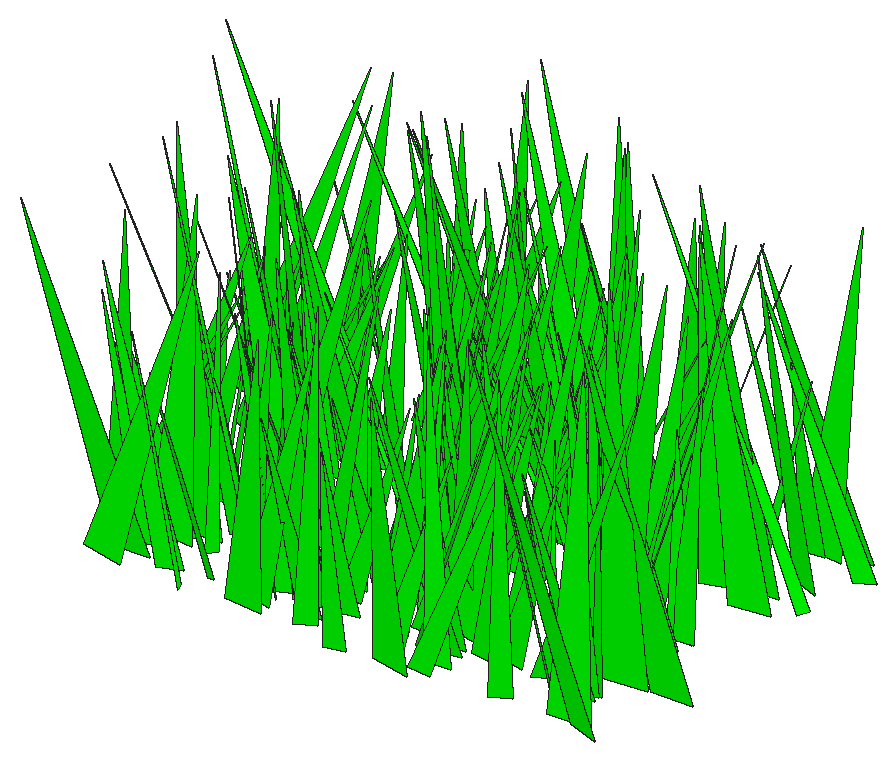
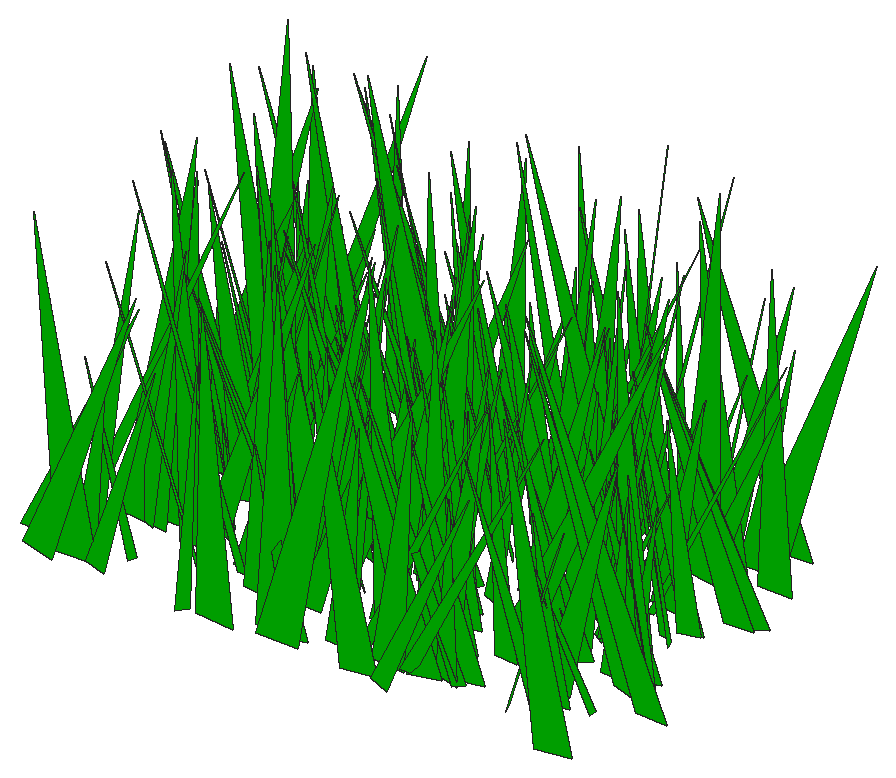
# SketchUp Ruby script. Lengths in inches.
U = 1.inch
M = Sketchup.active_model
def pt(a) = Geom::Point3d.new(a.map { |v| v * U })
def face(e, loops, mat)
  f = e.add_face(loops[0].map { |a| pt(a) })
  loops[1..].each { |l| e.add_face(l.map { |a| pt(a) }).erase! }
  f.material = f.back_material = mat if mat
  f
end
# faces: each face lists its corners as indices into pts; further lists are holes
def faces(e, pts, list, mat = nil) = list.each { |f| face(e, (f[0].is_a?(Array) ? f : [f]).map { |l| l.map { |i| pts[i] } }, mat) }
# xy, xz, yz: faces in a plane at the given z, y or x. An outline is a flat list of corners, or four numbers for a rectangle; further outlines are holes
def ring(l) = l.size == 4 ? [[l[0], l[1]], [l[2], l[1]], [l[2], l[3]], [l[0], l[3]]] : l.each_slice(2).to_a
def flat(e, list, mat, &to3) = list.each { |f| face(e, (f[0].is_a?(Array) ? f : [f]).map { |l| ring(l).map { |u, v| to3.(u, v) } }, mat) }
def xy(e, z, list, mat = nil) = flat(e, list, mat) { |x, y| [x, y, z] }
def xz(e, y, list, mat = nil) = flat(e, list, mat) { |x, z| [x, y, z] }
def yz(e, x, list, mat = nil) = flat(e, list, mat) { |y, z| [x, y, z] }
def lines(e, pts, list) = list.each { |a, b| e.add_line(pt(pts[a]), pt(pts[b])) }
# prism: a flat outline (further loops are holes) pulled along v
def prism(e, loops, v, mat = nil)
  f = face(e, loops, mat); d = Geom::Vector3d.new(v.map { |x| x * U })
  f.pushpull(f.normal.samedirection?(d) ? d.length : -d.length)
end
def box(e, o, s, mat = nil) = prism(e, [[o, [o[0] + s[0], o[1], o[2]], [o[0] + s[0], o[1] + s[1], o[2]], [o[0], o[1] + s[1], o[2]]]], [0, 0, s[2]], mat)
def at(x, y, z, deg = 0) = Geom::Transformation.translation(pt([x, y, z])) * Geom::Transformation.rotation(ORIGIN, Z_AXIS, deg.degrees)
def axes(o, x, y, z) = Geom::Transformation.new([*x, 0, *y, 0, *z, 0, *pt(o).to_a, 1])
def part(name) = M.definitions.add(name)
# library, detail: a bought-in or finely detailed component or shape, given as its bounding box
def library(name, o, s) = part(name).tap { |d| box(d.entities, o, s) }
def detail(e, o, s) = box(e.add_group.entities, o, s)
def put(e, d, t, mat = nil) = e.add_instance(d, t).tap { |i| i.material = mat if mat }
def group(e, t, mat = nil) = e.add_group.tap { |g| g.transformation = t; g.material = mat if mat }.entities
root = M.entities
M.materials.add("[0065_Lime]").color = [0, 255, 0]
c1 = part("fur_instance\#9")
p = [[0.8125,0,1.79],[0.67,-0.02,1.48],[0,-0.11,0],[0,0.11,0]]
faces(c1.entities,p,[[0,1,2,3]])
put(root,c1,axes([91.92,19.48,1.48],[-3.24569,-1.02685,0.182],[7.276,-0.45031,0.71645],[-0.71502,0.07882,6.46446]),"[0065_Lime]")
put(root,c1,axes([92.61,24.42,1.48],[-7.02476,-0.26887,0.02908],[1.8862,-0.97596,-0.89575],[0.32351,-0.148,5.85407]),"[0065_Lime]")
put(root,c1,axes([89.58,28.3,1.48],[4.62409,0.12298,1.08018],[-0.66506,0.67068,-0.67486],[-1.44467,0.08487,3.76811]),"[0065_Lime]")
put(root,c1,axes([89.8,28.16,1.48],[3.69978,-0.35848,0.84872],[2.50533,0.5397,0.41241],[-1.14897,0.02248,3.63218]),"[0065_Lime]")
put(root,c1,axes([91.04,27.25,1.48],[-2.89217,0.42946,0.19512],[-3.00695,-0.40642,0.48535],[0.59731,0.03349,3.3881]),"[0065_Lime]")
put(root,c1,axes([89.41,33.39,1.48],[2.35109,-0.91741,1.43617],[6.76165,0.31301,-0.62389],[0.15009,0.26967,5.60987]),"[0065_Lime]")
put(root,c1,axes([91.9,30.17,1.48],[-2.7268,0.71224,1.12489],[-5.24775,-0.35859,-0.80864],[-0.25507,-0.23663,4.61131]),"[0065_Lime]")
put(root,c1,axes([90.42,20.89,1.48],[-2.77263,-0.88074,1.86179],[6.51417,-0.43273,-0.44095],[1.44572,0.26072,5.55742]),"[0065_Lime]")
put(root,c1,axes([88.35,29.73,1.48],[5.98614,0.89507,0.55434],[-6.40524,0.83845,0.39983],[-0.10668,-0.11712,7.09892]),"[0065_Lime]")
put(root,c1,axes([91.03,28.375,1.48],[1.26403,-0.5368,0.92286],[3.89497,0.20179,0.40328],[-0.84273,0.12746,3.24813]),"[0065_Lime]")
put(root,c1,axes([89.76,27.91,1.48],[3.22694,0.49716,0.9492],[-3.72481,0.43486,0.74612],[-0.07426,-0.20831,3.82301]),"[0065_Lime]")
put(root,c1,axes([92.01,20.15,1.48],[-3.96111,0.47657,1.19406],[-3.61441,-0.56262,-0.40871],[0.77039,-0.18925,4.22195]),"[0065_Lime]")
put(root,c1,axes([92.32,32.04,1.48],[-4.69595,-0.0008,0.64551],[0.12397,-0.66172,0.56935],[0.78386,0.09988,3.77708]),"[0065_Lime]")
put(root,c1,axes([90.81,24.77,1.48],[-2.10896,0.56806,1.28674],[-4.12646,-0.33907,0.54107],[1.34808,-0.14921,3.66919]),"[0065_Lime]")
put(root,c1,axes([92.78,21.3125,1.48],[-3.49706,0.4689,0.33335],[-3.35687,-0.48239,-0.56302],[-0.18611,-0.10996,3.89128]),"[0065_Lime]")
put(root,c1,axes([92.83,26.69,1.48],[-8.75074,-0.02631,1.80702],[-0.08493,-1.25958,-0.88654],[2.22778,-0.15135,7.06419]),"[0065_Lime]")
put(root,c1,axes([90.9,25.63,1.48],[4.04277,0.01574,1.04251],[0.11871,0.58679,-0.60154],[-1.28105,0.10406,3.23424]),"[0065_Lime]")
put(root,c1,axes([92.92,26.6875,1.48],[-3.81514,-0.23371,0.32544],[1.70696,-0.52916,0.50596],[0.11291,0.10271,3.34735]),"[0065_Lime]")
put(root,c1,axes([89.25,23.09,1.48],[5.133,-0.39887,0.1458],[2.83923,0.71551,-0.54425],[0.16811,0.09442,4.74]),"[0065_Lime]")
put(root,c1,axes([94.78,28.57,1.48],[-7.87068,0.70308,0.34183],[-5.02024,-1.0998,-0.67967],[-0.09552,-0.13074,7.55576]),"[0065_Lime]")
put(root,c1,axes([89.88,23.375,1.48],[3.25022,0.81752,0.41828],[-5.82461,0.44758,0.63277],[0.43207,-0.11612,5.38373]),"[0065_Lime]")
put(root,c1,axes([90,30.6,1.48],[4.06266,-0.08517,0.13062],[0.62466,0.56262,-0.56183],[-0.05456,0.09935,3.29362]),"[0065_Lime]")
put(root,c1,axes([91.54,26.5625,1.48],[3.93743,0.99503,1.61528],[-7.17486,0.58923,-0.59105],[-1.615,-0.19181,6.56394]),"[0065_Lime]")
put(root,c1,axes([91.58,26.08,1.48],[4.62297,0.14912,1.48012],[-0.79049,0.6944,-0.71064],[-1.95252,0.07193,3.79218]),"[0065_Lime]")
put(root,c1,axes([89.97,28.9375,1.48],[6.16256,0.78027,0.25446],[-5.49819,0.8646,-0.73643],[-0.83749,0.06533,6.70714]),"[0065_Lime]")
put(root,c1,axes([92.52,23.83,1.48],[0.18841,-0.66559,1.23709],[4.89414,0.06316,0.64558],[-0.89245,0.20587,3.80149]),"[0065_Lime]")
put(root,c1,axes([90.24,32.62,1.48],[4.00656,0.60155,0.63818],[-4.35167,0.55614,0.51018],[-0.07102,-0.14079,4.74197]),"[0065_Lime]")
put(root,c1,axes([91.14,30.91,1.48],[0.02874,-0.59972,0.24403],[4.21195,-0.00344,-0.61147],[0.75158,0.04221,3.41741]),"[0065_Lime]")
put(root,c1,axes([90.77,24.6,1.48],[3.40058,0.61504,0.9237],[-4.51374,0.47364,0.42691],[-0.27052,-0.17163,4.48824]),"[0065_Lime]")
put(root,c1,axes([89.79,22.42,1.48],[5.33353,0.25038,0.28486],[-1.81571,0.73758,0.76943],[-0.02711,-0.14168,4.50888]),"[0065_Lime]")
put(root,c1,axes([91.4,25.32,1.48],[4.15817,-0.09228,0.84533],[0.5224,0.59889,0.49051],[-1.11283,-0.06367,3.38892]),"[0065_Lime]")
put(root,c1,axes([93.59,19.34,1.48],[3.44491,-0.59274,2.93219],[4.61273,0.6373,0.73132],[-3.08396,0.29112,4.36922]),"[0065_Lime]")
put(root,c1,axes([92.99,27.52,1.48],[0.50021,0.56005,0.98968],[-4.05679,0.10481,-0.63089],[-0.95276,-0.15226,3.20588]),"[0065_Lime]")
put(root,c1,axes([92.96,21.65,1.48],[2.47919,1.16013,2.39013],[-8.58156,0.40836,-0.75235],[-1.7761,-0.35368,6.9714]),"[0065_Lime]")
put(root,c1,axes([92.32,20.95,1.48],[-1.36073,1.04462,1.98532],[-7.74686,-0.22878,0.52058],[1.09942,-0.31913,6.12535]),"[0065_Lime]")
put(root,c1,axes([93.99,25.67,1.48],[-5.63766,-0.40911,1.36757],[3.13367,-0.80652,0.46238],[1.21799,0.18139,5.14041]),"[0065_Lime]")
put(root,c1,axes([93.57,27.14,1.48],[0.24656,0.87384,0.72564],[-6.21892,0.05173,-0.68939],[-0.89053,-0.11932,5.01518]),"[0065_Lime]")
put(root,c1,axes([93.65,26.5,1.48],[-7.34357,-0.52266,1.95346],[3.62738,-1.085,-0.7053],[2.53863,0.03841,6.65863]),"[0065_Lime]")
put(root,c1,axes([94.04,22.4375,1.48],[0.02603,-0.59967,1.14393],[4.35653,0.05176,0.84369],[-1.10039,0.19075,3.3673]),"[0065_Lime]")
put(root,c1,axes([91.3125,18.75,1.48],[3.56995,0.98302,0.75879],[-7.048,0.48889,0.71644],[0.36871,-0.17267,6.3482]),"[0065_Lime]")
put(root,c1,axes([94.92,24.03,1.48],[-3.06708,1.05085,0.18006],[-7.46739,-0.42789,-0.48009],[-0.46251,-0.06018,6.55721]),"[0065_Lime]")
put(root,c1,axes([93.96,26.22,1.48],[-0.35939,-0.56633,0.89823],[4.13365,-0.02534,0.55892],[-0.61279,0.1612,3.24348]),"[0065_Lime]")
put(root,c1,axes([96.28,32.16,1.48],[-6.77188,0.27227,0.21489],[-1.95548,-0.94195,-0.7813],[-0.0128,-0.13997,5.67585]),"[0065_Lime]")
put(root,c1,axes([93.1,24.56,1.48],[3.48195,-0.26171,1.27705],[2.25104,0.49277,-0.67705],[-0.9308,0.2127,3.13981]),"[0065_Lime]")
put(root,c1,axes([94.58,18.6,1.48],[-5.3622,-0.02784,1.16169],[0.04171,-0.77552,-0.4953],[1.44123,-0.08112,4.33646]),"[0065_Lime]")
put(root,c1,axes([95,19.66,1.48],[-4.02091,-0.1927,0.537],[1.4559,-0.56336,0.43859],[0.44365,0.10228,3.4277]),"[0065_Lime]")
put(root,c1,axes([92.29,28.17,1.48],[4.68915,-0.38873,0.81739],[2.92828,0.64294,-0.86891],[-0.29672,0.20182,4.34245]),"[0065_Lime]")
put(root,c1,axes([92.98,28.25,1.48],[3.17941,-0.50135,1.25079],[3.87054,0.43291,-0.69516],[-0.33628,0.24265,3.82459]),"[0065_Lime]")
put(root,c1,axes([95.95,20.75,1.48],[-9.06066,0.02591,1.57194],[-0.0697,-1.2997,0.45217],[1.94005,0.07434,7.3577]),"[0065_Lime]")
put(root,c1,axes([93.97,21,1.48],[5.84968,-0.28453,1.8218],[1.88023,0.88016,0.61173],[-2.36242,-0.00402,4.9979]),"[0065_Lime]")
put(root,c1,axes([96.45,33.36,1.48],[-3.92188,-0.48157,0.54721],[3.48617,-0.53123,0.86575],[-0.21028,0.17445,4.14707]),"[0065_Lime]")
put(root,c1,axes([96.13,26.02,1.48],[2.66254,0.7062,3.1752],[-5.72082,0.52604,-0.74642],[-2.78699,-0.40513,4.56559]),"[0065_Lime]")
put(root,c1,axes([94.69,23.99,1.48],[-3.47755,-0.55923,1.54151],[4.09865,-0.53505,-0.38659],[1.62212,0.15303,4.28154]),"[0065_Lime]")
put(root,c1,axes([94.98,31.8125,1.48],[1.89635,0.58542,0.48265],[-4.0538,0.27867,-0.7882],[-1.12956,-0.01729,3.63899]),"[0065_Lime]")
put(root,c1,axes([94.32,29.62,1.48],[3.96928,-0.50861,0.78173],[3.52731,0.57385,0.66095],[-1.25816,0.00424,4.31923]),"[0065_Lime]")
put(root,c1,axes([95.62,31.26,1.48],[-3.60186,-0.89989,0.59524],[6.39015,-0.51395,-0.45239],[0.84485,0.05087,5.95941]),"[0065_Lime]")
put(root,c1,axes([94.9,22.94,1.48],[4.65332,0.1835,1.54487],[-1.66986,0.68285,0.61007],[-1.58872,-0.18026,3.88367]),"[0065_Lime]")
put(root,c1,axes([94.21,31.46,1.48],[1.35391,0.67375,1.23494],[-4.97952,0.14855,0.89635],[0.70629,-0.24421,3.95224]),"[0065_Lime]")
put(root,c1,axes([96.59,23.53,1.48],[-2.92017,0.39625,1.0527],[-3.09301,-0.3915,-0.73886],[0.24508,-0.21949,3.2183]),"[0065_Lime]")
put(root,c1,axes([98.27,31.92,1.48],[-6.97872,0.18079,0.44711],[-1.35547,-0.97103,-0.84115],[0.34673,-0.15718,5.71063]),"[0065_Lime]")
put(root,c1,axes([98.65,21.36,1.48],[-7.58601,-0.24268,0.39256],[1.75768,-1.06469,0.41787],[0.35528,0.08554,6.31464]),"[0065_Lime]")
put(root,c1,axes([95.74,31.46,1.48],[2.89192,-0.97652,1.20471],[7.01807,0.42769,0.47013],[-1.11118,0.15977,6.10459]),"[0065_Lime]")
put(root,c1,axes([97,26.9375,1.48],[-4.809,-0.40122,1.63168],[3.26029,-0.68769,0.69141],[1.24379,0.25134,4.49638]),"[0065_Lime]")
put(root,c1,axes([97.2,28.99,1.48],[-4.79847,-0.58684,0.55181],[4.05876,-0.67916,-0.85042],[1.19503,-0.04971,5.10404]),"[0065_Lime]")
put(root,c1,axes([97.34,20.45,1.48],[3.29526,-0.56739,2.37379],[4.25461,0.5763,0.708],[-2.5921,0.22461,4.17981]),"[0065_Lime]")
put(root,c1,axes([97.23,20.11,1.48],[-8.2028,-0.2169,2.21285],[1.39841,-1.21403,-0.55761],[2.79783,-0.02911,6.76643]),"[0065_Lime]")
put(root,c1,axes([95.75,29.83,1.48],[3.9972,0.6986,0.67111],[-4.93396,0.57262,-0.5301],[-1.0264,-0.03202,5.16178]),"[0065_Lime]")
put(root,c1,axes([94.43,31.84,1.48],[6.13335,-0.25662,0.59584],[1.8984,0.86035,-0.51303],[-0.51748,0.11473,5.18006]),"[0065_Lime]")
put(root,c1,axes([97.01,32.21,1.48],[1.35334,-0.78828,1.09447],[5.68313,0.21554,0.55238],[-0.99121,0.15954,4.66139]),"[0065_Lime]")
put(root,c1,axes([96.17,20.04,1.48],[-3.0635,-0.7169,2.06526],[5.32815,-0.50401,-0.63327],[2.02148,0.24201,4.799]),"[0065_Lime]")
put(root,c1,axes([96.41,28.73,1.48],[-2.88419,-0.55562,1.77818],[4.03701,-0.48056,-0.6993],[2.02893,0.16635,3.91914]),"[0065_Lime]")
put(root,c1,axes([97.02,27.95,1.48],[4.01211,-0.20807,1.20173],[1.31206,0.60007,0.58326],[-1.62906,-0.02915,3.42943]),"[0065_Lime]")
put(root,c1,axes([96.43,29.51,1.48],[4.03494,0.59472,0.31955],[-4.14039,0.56714,-0.77818],[-0.96142,0.05355,4.69237]),"[0065_Lime]")
put(root,c1,axes([95.11,22.55,1.48],[7.41351,-0.70839,1.27092],[5.18238,1.04872,-0.41399],[-0.99944,0.18329,7.28065]),"[0065_Lime]")
put(root,c1,axes([96.41,29.53,1.48],[-0.01607,-0.59195,0.6162],[4.15328,-0.02789,-0.82607],[1.03465,0.10275,3.32558]),"[0065_Lime]")
put(root,c1,axes([98.6,30.34,1.48],[-4.83189,-0.82478,1.6828],[6.17604,-0.68084,0.55145],[0.76717,0.28629,6.1594]),"[0065_Lime]")
put(root,c1,axes([98.72,22.33,1.48],[-5.0712,0.17989,0.7661],[-1.38387,-0.71742,-0.41608],[0.78159,-0.10305,4.234]),"[0065_Lime]")
put(root,c1,axes([96.88,18.93,1.48],[0.07756,-0.90827,0.96952],[6.55338,-0.00216,-0.41461],[0.50402,0.16783,5.24171]),"[0065_Lime]")
put(root,c1,axes([96.87,29.85,1.48],[0.23418,0.58236,1.02324],[-4.30254,0.01099,0.44191],[0.49642,-0.17947,3.34742]),"[0065_Lime]")
put(root,c1,axes([95.63,32.08,1.48],[4.04911,-0.82869,0.45845],[5.91356,0.5596,-0.66201],[0.35608,0.1298,5.78109]),"[0065_Lime]")
put(root,c1,axes([98.43,20.34,1.48],[3.146,0.86777,2.32926],[-6.42121,0.52544,-0.82127],[-2.25938,-0.28503,5.57735]),"[0065_Lime]")
put(root,c1,axes([97.43,27.34,1.48],[-3.77375,0.12988,1.78464],[-0.69374,-0.61272,0.52366],[2.27745,0.02858,3.11667]),"[0065_Lime]")
put(root,c1,axes([97.27,23.65,1.48],[0.06631,0.84537,0.371],[-5.98966,0.00152,0.59219],[0.72509,-0.06475,4.85793]),"[0065_Lime]")
put(root,c1,axes([97.73,30.89,1.48],[3.76272,1.15651,1.00381],[-8.19997,0.54771,-0.80828],[-1.4221,-0.09816,7.31663]),"[0065_Lime]")
put(root,c1,axes([96.86,19.53,1.48],[3.13879,0.7728,1.39934],[-5.76187,0.4247,0.6919],[-0.07946,-0.26944,5.10409]),"[0065_Lime]")
put(root,c1,axes([98.94,19.74,1.48],[-0.671,-0.6326,0.24657],[4.47151,-0.08747,0.53171],[-0.60374,0.05526,3.66397]),"[0065_Lime]")
put(root,c1,axes([99.13,27.23,1.48],[3.53624,1.04666,3.01769],[-7.90001,0.60022,-0.85075],[-2.6143,-0.39801,6.65272]),"[0065_Lime]")
put(root,c1,axes([97.19,27.82,1.48],[2.91879,0.6709,0.89423],[-4.89693,0.40524,0.38767],[-0.15692,-0.16692,4.53533]),"[0065_Lime]")
put(root,c1,axes([99.05,21.11,1.48],[-5.98973,0.45164,2.31292],[-3.83022,-0.87203,-0.85691],[1.93532,-0.32803,5.46246]),"[0065_Lime]")
put(root,c1,axes([97.45,33.16,1.48],[0.67535,0.89881,2.10819],[-6.86108,0.04787,0.7704],[0.74631,-0.3733,5.17481]),"[0065_Lime]")
put(root,c1,axes([99.23,27.38,1.48],[-6.73477,-0.69264,1.98789],[5.01224,-0.99626,-0.3965],[2.26872,0.14488,6.77708]),"[0065_Lime]")
put(root,c1,axes([101,23.42,1.48],[-6.17188,0.12817,0.08532],[-0.89091,-0.86023,0.66272],[0.22201,0.11113,5.03136]),"[0065_Lime]")
put(root,c1,axes([98.13,26.65,1.48],[3.85492,-0.13487,0.78219],[0.83073,0.55564,0.50159],[-1.07511,-0.05426,3.19221]),"[0065_Lime]")
put(root,c1,axes([98.99,32.16,1.48],[1.25087,-0.68207,0.7598],[4.87414,0.19272,0.48801],[-0.8224,0.10479,4.04797]),"[0065_Lime]")
put(root,c1,axes([101.65,29.14,1.48],[-5.65504,-0.91894,0.24835],[6.5208,-0.78557,0.83936],[-0.58275,0.12712,6.98219]),"[0065_Lime]")
put(root,c1,axes([98.76,22.14,1.48],[-1.56191,0.72731,0.5264],[-5.15281,-0.22989,0.52752],[0.81092,-0.05991,4.36593]),"[0065_Lime]")
put(root,c1,axes([100.75,33.14,1.48],[-5.09117,0.98867,0.97003],[-7.12989,-0.71342,-0.3938],[0.3021,-0.1758,7.05329]),"[0065_Lime]")
put(root,c1,axes([99.73,20.54,1.48],[0.21944,-0.71584,1.10892],[5.19335,0.06265,0.67523],[-0.91637,0.18364,4.09229]),"[0065_Lime]")
put(root,c1,axes([99.99,30.3,1.48],[-7.25894,-0.28331,2.29608],[2.47774,-1.06729,0.76994],[2.42774,0.24217,6.07948]),"[0065_Lime]")
put(root,c1,axes([98.27,24.32,1.48],[4.82662,0.10074,0.65315],[-0.53372,0.67411,-0.87433],[-0.9348,0.13524,3.87161]),"[0065_Lime]")
put(root,c1,axes([99.17,19.22,1.48],[6.00487,-0.56016,1.82566],[3.95589,0.89718,0.61538],[-2.29783,0.08071,5.8304]),"[0065_Lime]")
put(root,c1,axes([101.3125,30.86,1.48],[-4.0096,0.58161,0.46494],[-4.17832,-0.55757,-0.46903],[-0.02049,-0.11405,4.66395]),"[0065_Lime]")
put(root,c1,axes([100.71,21.65,1.48],[-0.04136,-0.70623,0.08517],[4.91148,-0.00254,0.87209],[-1.07149,0.01561,3.99418]),"[0065_Lime]")
put(root,c1,axes([98.77,20.62,1.48],[-5.2944,-0.58766,3.22173],[4.40357,-0.90025,-0.71452],[3.71299,0.22973,5.44132]),"[0065_Lime]")
put(root,c1,axes([101.37,30.6875,1.48],[-6.69287,0.05615,1.49717],[-0.71159,-0.95938,-0.89908],[1.74389,-0.17598,5.37914]),"[0065_Lime]")
put(root,c1,axes([102.23,30.4,1.48],[-6.22703,0.97138,0.22501],[-6.88805,-0.87537,0.50627],[0.64738,0.02974,7.55102]),"[0065_Lime]")
put(root,c1,axes([102.09,28.44,1.48],[-4.57817,0.0141,0.06638],[-0.1099,-0.6382,-0.4719],[0.06821,-0.08176,3.69483]),"[0065_Lime]")
put(root,c1,axes([99.29,29.02,1.48],[3.67206,0.71727,1.24036],[-5.31064,0.51348,0.45244],[-0.42237,-0.22023,5.09476]),"[0065_Lime]")
put(root,c1,axes([99.23,21.4,1.48],[3.65346,-0.46943,0.82904],[3.4828,0.50527,-0.56798],[-0.26356,0.16961,3.98661]),"[0065_Lime]")
put(root,c1,axes([100.07,22.29,1.48],[3.58474,0.46932,0.514],[-3.20099,0.5095,-0.81802],[-1.14371,0.04501,3.90049]),"[0065_Lime]")
put(root,c1,axes([97.95,26.51,1.48],[7.68545,-0.19898,0.63195],[1.48887,1.07853,-0.60092],[-0.62611,0.12229,6.3282]),"[0065_Lime]")
put(root,c1,axes([99.55,23.67,1.48],[-3.176,-0.44217,2.04305],[3.05681,-0.55738,-0.89815],[2.62036,0.11429,3.52402]),"[0065_Lime]")
put(root,c1,axes([100.87,18.57,1.48],[1.84091,-0.55287,0.9926],[3.98598,0.28648,0.45583],[-1.04005,0.11935,3.50387]),"[0065_Lime]")
put(root,c1,axes([99.44,26.61,1.48],[7.19532,0.51889,2.065],[-4.08172,1.03739,0.67527],[-1.8494,-0.2708,6.54377]),"[0065_Lime]")
put(root,c1,axes([101.19,32.6,1.48],[-3.44879,1.00705,1.58353],[-7.30548,-0.51427,0.43196],[1.33494,-0.21264,6.45495]),"[0065_Lime]")
put(root,c1,axes([99.52,26.02,1.48],[2.31844,-0.59017,0.22756],[4.14684,0.31254,-0.79284],[0.7224,0.1,3.82088]),"[0065_Lime]")
put(root,c1,axes([100.26,32.76,1.48],[0.23878,-0.54852,1.10261],[4.03808,-0.00953,-0.73744],[0.87721,0.19317,3.09452]),"[0065_Lime]")
put(root,c1,axes([101.77,22.9,1.48],[-0.23271,0.92191,0.64966],[-6.58665,-0.02307,-0.46413],[-0.54624,-0.1146,5.31981]),"[0065_Lime]")
put(root,c1,axes([100.68,22.49,1.48],[-0.01571,0.81854,1.26315],[-5.99652,-0.0246,0.48491],[0.62112,-0.21683,4.7134]),"[0065_Lime]")
put(root,c1,axes([102.65,28.29,1.48],[-5.45352,-0.84059,1.64861],[6.24494,-0.77393,0.44529],[0.94529,0.26341,6.56935]),"[0065_Lime]")
put(root,c1,axes([102.05,25.9375,1.48],[-1.10696,0.691,0.74359],[-4.99459,-0.14565,-0.38414],[-0.26837,-0.13958,4.08205]),"[0065_Lime]")
put(root,c1,axes([100.7,28.83,1.48],[3.97803,0.16264,0.42914],[-1.02369,0.55382,-0.75481],[-0.75504,0.10603,3.28435]),"[0065_Lime]")
put(root,c1,axes([101.12,24.09,1.48],[3.49977,0.40202,0.29265],[-2.73845,0.48829,-0.80898],[-0.90318,0.07733,3.58684]),"[0065_Lime]")
put(root,c1,axes([100.14,24.06,1.48],[8.62324,0.16471,1.72476],[-1.32436,1.24285,0.40388],[-2.02881,-0.11122,7.06723]),"[0065_Lime]")
put(root,c1,axes([102.42,23.2,1.48],[0.08837,0.68836,0.95847],[-5.00202,0.03187,-0.46173],[-0.60484,-0.16296,3.9585]),"[0065_Lime]")
put(root,c1,axes([102.05,27.11,1.48],[2.39831,0.50673,0.09199],[-3.48865,0.33057,-0.839],[-0.91997,0.06744,3.42139]),"[0065_Lime]")
put(root,c1,axes([101.91,21.8,1.48],[5.97637,-0.22166,2.131],[2.01129,0.89367,-0.61718],[-2.3036,0.2052,4.98972]),"[0065_Lime]")
put(root,c1,axes([104.02,20.55,1.48],[-4.01416,-0.57477,0.89186],[4.23475,-0.54402,0.86265],[-0.01595,0.21434,4.58118]),"[0065_Lime]")
put(root,c1,axes([104.14,27.9,1.48],[-3.83485,-0.3415,0.30394],[2.4501,-0.52249,0.78146],[-0.20754,0.14188,3.60935]),"[0065_Lime]")
put(root,c1,axes([101.45,20.75,1.48],[3.47663,0.85199,1.53017],[-6.33236,0.4868,0.43673],[-0.45062,-0.2675,5.66837]),"[0065_Lime]")
put(root,c1,axes([102.85,31.16,1.48],[2.66331,1.05933,1.93104],[-7.76446,0.41647,-0.57031],[-1.47735,-0.27909,6.47852]),"[0065_Lime]")
put(root,c1,axes([103.07,22.67,1.48],[-2.58882,-0.63951,0.23267],[4.49639,-0.36569,-0.5787],[0.75944,-0.01489,4.21943]),"[0065_Lime]")
put(root,c1,axes([102.38,30.65,1.48],[-5.38241,-0.84504,2.57452],[6.14859,-0.84719,-0.81288],[2.89445,0.22825,6.51426]),"[0065_Lime]")
put(root,c1,axes([102.98,18.74,1.48],[-2.03752,-0.92539,0.12117],[6.53216,-0.28667,-0.68636],[0.84999,-0.01521,5.56513]),"[0065_Lime]")
put(root,c1,axes([103.67,20.98,1.48],[-0.73871,-0.74986,1.05637],[5.47816,-0.08747,0.4541],[-0.39172,0.19086,4.35849]),"[0065_Lime]")
put(root,c1,axes([103.39,30.36,1.48],[2.63272,0.94834,1.65151],[-6.87582,0.41247,-0.68443],[-1.54698,-0.21937,5.85268]),"[0065_Lime]")
put(root,c1,axes([102.07,20,1.48],[1.69388,0.64425,0.27951],[-4.58141,0.23219,0.43676],[0.38655,-0.07123,3.95168]),"[0065_Lime]")
put(root,c1,axes([102.21,25.03,1.48],[2.94807,0.53939,0.99148],[-4.01448,0.41061,0.41249],[-0.3236,-0.17985,3.91529]),"[0065_Lime]")
put(root,c1,axes([104.24,30.24,1.48],[-0.74997,0.68554,1.17064],[-5.0122,-0.06478,-0.85336],[-0.86644,-0.21865,3.92327]),"[0065_Lime]")
put(root,c1,axes([103.4375,27.51,1.48],[-3.62563,0.37105,1.13579],[-2.61389,-0.54346,0.42857],[1.44575,-0.05204,3.62316]),"[0065_Lime]")
put(root,c1,axes([103.22,21.95,1.48],[-3.49713,-0.76158,1.86047],[5.56833,-0.54914,-0.60715],[1.89722,0.20791,5.21137]),"[0065_Lime]")
put(root,c1,axes([103.07,33.4,1.48],[2.92682,-0.92936,0.13218],[6.57981,0.41151,0.55511],[-0.6897,-0.01803,5.85679]),"[0065_Lime]")
put(root,c1,axes([102.76,28.42,1.48],[0.80048,0.95404,1.60072],[-7.03915,0.08206,0.69027],[0.64835,-0.28703,5.51791]),"[0065_Lime]")
put(root,c1,axes([104.07,19.79,1.48],[5.12374,-0.48293,2.99449],[4.27694,0.8069,-0.48145],[-2.65927,0.36727,4.99529]),"[0065_Lime]")
put(root,c1,axes([104.32,33.46,1.48],[-5.14227,0.32701,1.34956],[-2.16441,-0.75897,0.70592],[1.86653,0.02082,4.53661]),"[0065_Lime]")
put(root,c1,axes([102.2,25.97,1.48],[5.08179,0.57849,0.57673],[-4.17316,0.7101,0.46202],[-0.1892,-0.12486,5.2997]),"[0065_Lime]")
put(root,c1,axes([102.77,20.38,1.48],[6.3305,0.05353,0.87463],[-0.24876,0.89626,-0.64688],[-1.1133,0.10413,5.11791]),"[0065_Lime]")
put(root,c1,axes([103.16,21.8,1.48],[2.1432,1.21374,1.30258],[-8.77271,0.28356,0.69655],[0.46061,-0.24683,7.2054]),"[0065_Lime]")
put(root,c1,axes([101.99,24.82,1.48],[5.67175,-0.14309,0.01428],[1.00276,0.78215,-0.89762],[0.17805,0.15305,4.60049]),"[0065_Lime]")
put(root,c1,axes([102.39,21.2,1.48],[7.3818,0.73419,0.47632],[-5.16737,1.03929,-0.69418],[-0.96991,0.05076,7.32353]),"[0065_Lime]")
put(root,c1,axes([103.4,25.72,1.48],[7.10004,-0.10412,1.57043],[0.96785,1.02464,-0.61885],[-1.8275,0.13815,5.77356]),"[0065_Lime]")
put(root,c1,axes([106.7,28.77,1.48],[-5.8537,-0.64418,1.1221],[4.76284,-0.81458,0.76959],[0.48394,0.225,5.99869]),"[0065_Lime]")
put(root,c1,axes([104.36,27.85,1.48],[-5.41949,-0.63662,3.72717],[5.63964,-0.87559,0.41427],[3.11703,0.47734,5.73078]),"[0065_Lime]")
put(root,c1,axes([102.82,29.41,1.48],[6.87189,-0.09531,0.0944],[0.66357,0.96117,0.55648],[-0.18213,-0.09409,5.58921]),"[0065_Lime]")
put(root,c1,axes([104.81,21.05,1.48],[6.70792,0.58519,1.65739],[-4.15787,0.98209,-0.48523],[-2.0511,-0.07704,6.40397]),"[0065_Lime]")
put(root,c1,axes([104.28,23.5,1.48],[8.37978,-0.53519,1.34545],[3.68966,1.19984,0.78825],[-1.90487,-0.03031,7.44563]),"[0065_Lime]")
put(root,c1,axes([103.87,19.09,1.48],[6.32905,0.6618,0.14427],[-4.69185,0.88867,-0.41479],[-0.44649,0.04265,6.4037]),"[0065_Lime]")
put(root,c1,axes([104.37,28.15,1.48],[3.93993,-0.54193,0.27951],[3.84403,0.53921,-0.81898],[0.46424,0.13451,4.40922]),"[0065_Lime]")
put(root,c1,axes([104.35,32.24,1.48],[6.88875,0.05406,0.69537],[-0.44846,0.97235,0.40646],[-0.82323,-0.07732,5.59739]),"[0065_Lime]")
put(root,c1,axes([106.625,25.23,1.48],[-3.74738,-0.37024,1.29227],[2.61908,-0.56848,-0.43256],[1.61456,0.06283,3.70103]),"[0065_Lime]")
put(root,c1,axes([108.09,23.23,1.48],[-4.11346,0.35315,0.6765],[-2.64115,-0.56212,-0.79279],[0.17939,-0.17827,3.84003]),"[0065_Lime]")
put(root,c1,axes([104.32,30.45,1.48],[8.12595,-0.07928,0.83464],[0.43804,1.14331,0.81727],[-1.08595,-0.13205,6.57507]),"[0065_Lime]")
put(root,c1,axes([105.72,21.36,1.48],[0.6473,-0.61372,1.0482],[4.47211,0.0512,-0.82272],[0.85836,0.19606,3.49596]),"[0065_Lime]")
put(root,c1,axes([106.64,22.36,1.48],[-4.47883,0.08544,1.85501],[-0.95141,-0.69442,-0.44809],[2.15994,-0.1287,3.64915]),"[0065_Lime]")
put(root,c1,axes([106.92,19.37,1.48],[5.7454,-0.54821,2.03869],[3.89718,0.87474,0.61516],[-2.51282,0.1032,5.61539]),"[0065_Lime]")
put(root,c1,axes([108.19,33.03,1.48],[-3.35125,-0.50574,0.86732],[3.74794,-0.46199,0.55464],[0.20897,0.17541,3.96156]),"[0065_Lime]")
put(root,c1,axes([108.71,23.94,1.48],[-6.7716,0.07307,0.94692],[-0.36347,-0.95801,0.75733],[1.22209,0.11994,5.47217]),"[0065_Lime]")
put(root,c1,axes([107.61,21.33,1.48],[-3.87349,-0.18179,0.83363],[1.18306,-0.56199,-0.4695],[1.15083,-0.03415,3.28849]),"[0065_Lime]")
put(root,c1,axes([108.4,20.21,1.48],[-5.64334,-0.04536,0.95254],[0.43838,-0.80534,0.43332],[1.13286,0.08568,4.57741]),"[0065_Lime]")
put(root,c1,axes([106.45,29.96,1.48],[-2.94486,-1.01021,2.22854],[7.40375,-0.48419,-0.88155],[2.09178,0.29156,6.2576]),"[0065_Lime]")
put(root,c1,axes([108.08,23.12,1.48],[-1.07142,0.87763,1.2838],[-6.42132,-0.12748,-0.62555],[-0.51625,-0.2358,5.11645]),"[0065_Lime]")
put(root,c1,axes([108.87,25.04,1.48],[-2.20949,0.86179,0.19994],[-6.07785,-0.30207,-0.81091],[-0.85625,-0.07963,5.24011]),"[0065_Lime]")
put(root,c1,axes([106.56,24.83,1.48],[-0.73783,1.14968,1.49636],[-8.31228,-0.1346,0.75356],[1.10969,-0.24383,6.63953]),"[0065_Lime]")
put(root,c1,axes([108.27,25.49,1.48],[-5.46978,0.15695,1.36053],[-1.33034,-0.7931,-0.47293],[1.50846,-0.13033,4.51631]),"[0065_Lime]")
put(root,c1,axes([107.73,29.28,1.48],[5.26069,-0.75314,2.52429],[5.58659,0.82403,0.53513],[-2.67348,0.23995,6.08533]),"[0065_Lime]")
put(root,c1,axes([108.24,23.11,1.48],[0.61931,0.92603,0.84687],[-6.60945,0.10521,-0.65685],[-0.91054,-0.13382,5.34391]),"[0065_Lime]")
put(root,c1,axes([106.93,26.7,1.48],[-1.10316,0.92421,1.69337],[-6.76615,-0.20275,0.79163],[1.34616,-0.26171,5.36661]),"[0065_Lime]")
put(root,c1,axes([106.28,28.35,1.48],[8.1845,0.10954,1.68569],[-0.93315,1.1819,0.4242],[-2.00788,-0.10279,6.67404]),"[0065_Lime]")
put(root,c1,axes([109.07,21,1.48],[-2.79462,-0.53919,0.68836],[3.92832,-0.38001,0.57784],[-0.09069,0.15473,3.81776]),"[0065_Lime]")
put(root,c1,axes([108.84,29.74,1.48],[-5.27953,-0.45738,1.7692],[3.65438,-0.75982,0.63303],[1.404,0.25777,5.00515]),"[0065_Lime]")
put(root,c1,axes([108.93,29.74,1.48],[-1.26431,-1.24005,1.63778],[9.04009,-0.15854,0.59498],[-0.45772,0.29407,7.22712]),"[0065_Lime]")
put(root,c1,axes([111,29.59,1.48],[-9.04611,0.18186,0.73325],[-1.37774,-1.27012,-0.6903],[0.76773,-0.13648,7.40102]),"[0065_Lime]")
put(root,c1,axes([110.36,19.24,1.48],[-6.82091,-0.7348,0.37498],[5.17985,-0.95933,-0.65176],[0.85247,-0.05024,6.96064]),"[0065_Lime]")
put(root,c1,axes([109.58,28.66,1.48],[-2.74069,1.04318,1.36151],[-7.6097,-0.37293,-0.56054],[-0.08329,-0.25409,6.41253]),"[0065_Lime]")
put(root,c1,axes([110.27,33.34,1.48],[-3.60586,-0.8028,0.71735],[5.76349,-0.48796,0.86962],[-0.44699,0.18434,5.42609]),"[0065_Lime]")
put(root,c1,axes([107.2,24.69,1.48],[2.25984,-1.18304,1.44687],[8.59517,0.29796,-0.71847],[0.41191,0.273,7.05419]),"[0065_Lime]")
put(root,c1,axes([107.58,31.9,1.48],[4.10001,-0.13787,0.88191],[1.19213,0.5778,-0.64007],[-0.8468,0.14587,3.3689]),"[0065_Lime]")
put(root,c1,axes([108.86,32.78,1.48],[0.64705,-0.61026,0.60982],[4.35929,0.10427,0.43629],[-0.64784,0.09215,3.54485]),"[0065_Lime]")
put(root,c1,axes([109.02,21.26,1.48],[1.85283,0.53412,0.713],[-3.69788,0.28391,-0.76862],[-1.24181,-0.0485,3.35262]),"[0065_Lime]")
put(root,c1,axes([109.01,25.82,1.48],[-2.15824,0.60541,0.38027],[-4.27165,-0.30956,0.47369],[0.73097,-0.02148,3.89094]),"[0065_Lime]")
put(root,c1,axes([107.28,26.33,1.48],[5.2034,0.75424,1.11728],[-5.512,0.73154,0.43666],[-0.5617,-0.19161,6.06515]),"[0065_Lime]")
put(root,c1,axes([108.125,24.18,1.48],[4.65143,-0.04115,0.97851],[0.5769,0.65351,-0.89345],[-1.09548,0.16941,3.68424]),"[0065_Lime]")
put(root,c1,axes([111.31,32.3125,1.48],[-5.26332,0.52132,0.32805],[-3.72992,-0.73173,-0.63016],[-0.11997,-0.12157,5.19989]),"[0065_Lime]")
put(root,c1,axes([109.2,21.42,1.48],[-4.70658,-0.26953,2.05596],[2.36419,-0.72165,0.41082],[2.1162,0.20678,4.11364]),"[0065_Lime]")
put(root,c1,axes([109.96,30.95,1.48],[-5.71265,-0.66044,1.22477],[4.61456,-0.82955,-0.74849],[1.75034,0.03149,5.97061]),"[0065_Lime]")
put(root,c1,axes([107.16,21.2,1.48],[6.92484,-0.47103,0.51258],[3.32085,0.97681,0.39498],[-0.77835,-0.02312,6.24553]),"[0065_Lime]")
put(root,c1,axes([109.38,22.5,1.48],[2.50004,-1.21497,1.90786],[8.87284,0.3831,0.48228],[-1.23868,0.29201,7.30529]),"[0065_Lime]")
put(root,c1,axes([109.1,25.77,1.48],[2.82421,0.75088,0.47509],[-5.27353,0.40499,-0.7068],[-1.04189,-0.01449,4.86525]),"[0065_Lime]")
put(root,c1,axes([109.57,19.56,1.48],[1.39801,1.15468,0.14593],[-8.18885,0.19787,-0.55823],[-0.7067,-0.00859,6.75711]),"[0065_Lime]")
put(root,c1,axes([111.21,22.7,1.48],[-2.49928,-1.12899,0.38448],[8.02352,-0.34404,0.65655],[-0.63219,0.09687,6.81269]),"[0065_Lime]")
put(root,c1,axes([109.03,32.93,1.48],[1.26595,1.04395,1.50959],[-7.65434,0.16479,0.42847],[0.22381,-0.26925,6.11522]),"[0065_Lime]")
put(root,c1,axes([108.78,22.93,1.48],[5.68497,0.07873,0.73873],[-0.44229,0.80337,-0.61691],[-0.97113,0.09498,4.6055]),"[0065_Lime]")
